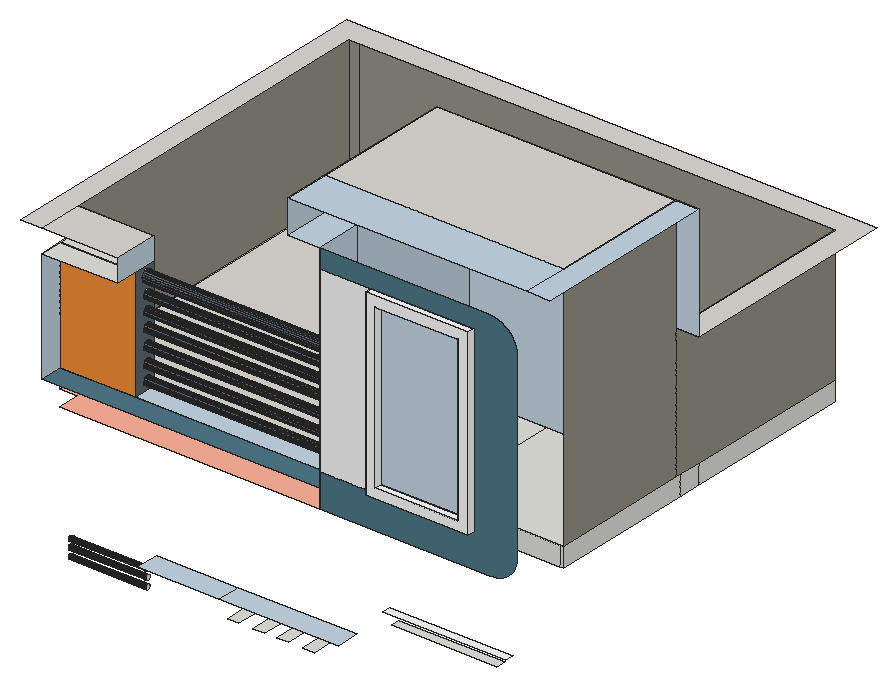
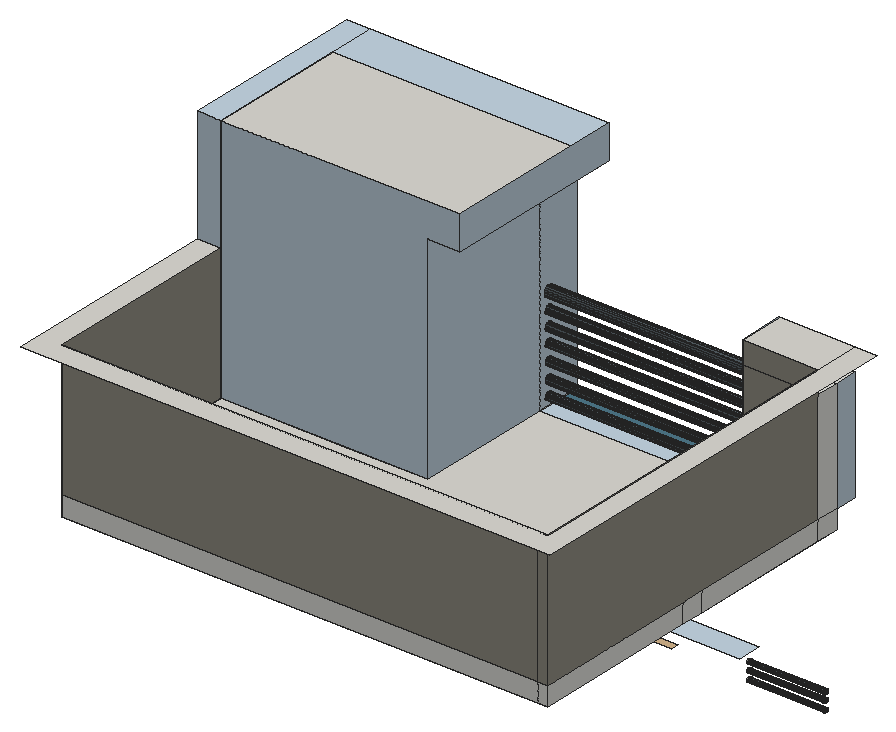
# SketchUp Ruby script. Lengths in inches.
U = 1.inch
M = Sketchup.active_model
def pt(a) = Geom::Point3d.new(a.map { |v| v * U })
def face(e, loops, mat)
  f = e.add_face(loops[0].map { |a| pt(a) })
  loops[1..].each { |l| e.add_face(l.map { |a| pt(a) }).erase! }
  f.material = f.back_material = mat if mat
  f
end
# faces: each face lists its corners as indices into pts; further lists are holes
def faces(e, pts, list, mat = nil) = list.each { |f| face(e, (f[0].is_a?(Array) ? f : [f]).map { |l| l.map { |i| pts[i] } }, mat) }
# xy, xz, yz: faces in a plane at the given z, y or x. An outline is a flat list of corners, or four numbers for a rectangle; further outlines are holes
def ring(l) = l.size == 4 ? [[l[0], l[1]], [l[2], l[1]], [l[2], l[3]], [l[0], l[3]]] : l.each_slice(2).to_a
def flat(e, list, mat, &to3) = list.each { |f| face(e, (f[0].is_a?(Array) ? f : [f]).map { |l| ring(l).map { |u, v| to3.(u, v) } }, mat) }
def xy(e, z, list, mat = nil) = flat(e, list, mat) { |x, y| [x, y, z] }
def xz(e, y, list, mat = nil) = flat(e, list, mat) { |x, z| [x, y, z] }
def yz(e, x, list, mat = nil) = flat(e, list, mat) { |y, z| [x, y, z] }
def lines(e, pts, list) = list.each { |a, b| e.add_line(pt(pts[a]), pt(pts[b])) }
# prism: a flat outline (further loops are holes) pulled along v
def prism(e, loops, v, mat = nil)
  f = face(e, loops, mat); d = Geom::Vector3d.new(v.map { |x| x * U })
  f.pushpull(f.normal.samedirection?(d) ? d.length : -d.length)
end
def box(e, o, s, mat = nil) = prism(e, [[o, [o[0] + s[0], o[1], o[2]], [o[0] + s[0], o[1] + s[1], o[2]], [o[0], o[1] + s[1], o[2]]]], [0, 0, s[2]], mat)
def at(x, y, z, deg = 0) = Geom::Transformation.translation(pt([x, y, z])) * Geom::Transformation.rotation(ORIGIN, Z_AXIS, deg.degrees)
def axes(o, x, y, z) = Geom::Transformation.new([*x, 0, *y, 0, *z, 0, *pt(o).to_a, 1])
def part(name) = M.definitions.add(name)
# library, detail: a bought-in or finely detailed component or shape, given as its bounding box
def library(name, o, s) = part(name).tap { |d| box(d.entities, o, s) }
def detail(e, o, s) = box(e.add_group.entities, o, s)
def put(e, d, t, mat = nil) = e.add_instance(d, t).tap { |i| i.material = mat if mat }
def group(e, t, mat = nil) = e.add_group.tap { |g| g.transformation = t; g.material = mat if mat }.entities
root = M.entities
M.materials.add("[0035_Tan]").color = [210, 180, 140]
M.materials.add("[0096_SkyBlue]").color = [79, 120, 137]
M.materials.add("[Blinds Vertical Pattern]").color = [247, 247, 249]
M.materials.add("[Cladding Siding Tan]").color = [242, 141, 55]
M.materials.add("[Color B02]").color = [255, 178, 153]
M.materials.add("[Formica Graystone]").color = [149, 146, 135]
M.materials.add("[Formica Speckled Grey]").color = [94, 105, 111]
M.materials.add("[Quartz Light Grey]").color = [251, 251, 252]
M.materials.add("[Terrazzo Light Blue]").color = [196, 214, 227]
M.materials.add("[Terrazzo Tile Light]").color = [219, 217, 210]
xy(root,314.29,[[158.09,175.18,164.38,187.5],[171.84,175.18,178.13,187.5],[184.46,175.18,190.75,187.5],[198.34,175.18,204.63,187.5]])
xy(root,322.125,[[110.1875,175.18,153.69,187.5],[153.69,175.18,217.34,187.5]],"[Terrazzo Light Blue]")
xy(root,354.33,[[259.5625,157.81,315.92,162.87]])
xy(root,358.97,[[254.93,157.81,320.55,162.87]],"[Quartz Light Grey]")
xy(root,372.97,[[81.24,265.26,131.93,269.39]],"[0035_Tan]")
xy(root,375.1875,[[158.92,265.26,207.48,270.7]],"[0035_Tan]")
xy(root,392.8125,[[68.53,265.26,328.05,277.89],[68.53,277.89,328.05,368.29]])
xy(root,392.8125,[[78.16,162.87,78.16,175.18,68.53,175.18,68.53,265.26,328.05,265.26,328.05,187.5,217.34,187.5,217.34,162.87]],"[Color B02]")
xy(root,403.0625,[[68.53,175.18,109.08,187.5],[217.34,187.5,259.37,262.25],[259.37,187.5,328.05,262.25]])
xy(root,403.0625,[[68.53,162.87,217.34,175.18]],"[0096_SkyBlue]")
xy(root,403.0625,[[109.08,175.18,217.34,187.5]],"[Terrazzo Light Blue]")
xy(root,403.0625,[[68.53,187.5,217.34,187.5,217.34,262.25,328.05,262.25,328.05,368.29,68.53,368.29]],"[Terrazzo Tile Light]")
xy(root,410.86,[[244.72,159.06,299.47,162.87]],"[Quartz Light Grey]")
xy(root,416.07,[[249.93,159.06,294.25,162.87]],"[Quartz Light Grey]")
xy(root,463,[[68.53,162.87,109.08,175.18],[68.53,175.18,109.08,187.5]])
xy(root,475.0625,[[57.16,162.87,68.53,162.87,68.53,368.29,328.05,368.29,328.05,262.25,340.49,262.25,340.49,380.73,57.16,380.73],[68.53,162.87,109.08,187.5]],"[Terrazzo Tile Light]")
xy(root,502.83,[[249.93,159.06,294.25,162.87]],"[Quartz Light Grey]")
xy(root,508.05,[[244.72,159.06,299.47,162.87]],"[Quartz Light Grey]")
xy(root,518.04,[[200.4,162.87,217.34,262.25]],"[Terrazzo Light Blue]")
xy(root,536.0625,[[200.4,162.87,328.05,187.5],[328.05,162.87,340.49,262.25]],"[Terrazzo Light Blue]")
xy(root,536.0625,[[200.4,187.5,328.05,262.25]],"[Terrazzo Tile Light]")
xz(root,159.06,[[[244.72,410.86,299.47,508.05],[249.93,416.07,294.25,502.83]]],"[Quartz Light Grey]")
xz(root,162.87,[[[244.72,410.86,299.47,508.05],[249.93,416.07,294.25,502.83]]])
xz(root,162.87,[[217.34,392.8125,308.15,392.8125,310.0625,392.92,311.9375,393.25,313.75,393.78,315.47,394.52,317.06,395.44,318.5,396.54,319.76,397.79,320.82,399.17,321.67,400.66,322.28,402.24,322.65,403.87,322.78,405.53,322.78,503.56,322.64,505.45,322.21,507.31,321.51,509.1,320.55,510.8,319.34,512.375,317.9,513.8,316.26,515.05,314.45,516.1,312.5,516.9375,310.4375,517.55,308.3,517.92,306.125,518.04,217.34,518.04,217.34,508.05,299.47,508.05,299.47,410.86,217.34,410.86]],"[0096_SkyBlue]")
xz(root,162.87,[[217.34,410.86,244.72,508.05]],"[Blinds Vertical Pattern]")
xz(root,162.87,[[249.93,416.07,294.25,502.83]],"[Terrazzo Light Blue]")
xz(root,175.18,[[68.53,403.0625,109.08,463]],"[Cladding Siding Tan]")
xz(root,187.5,[[217.34,392.8125,259.37,403.0625],[259.37,392.8125,326.14,403.0625],[326.14,392.8125,328.05,403.0625]])
xz(root,187.5,[[68.53,403.0625,109.08,463],[68.53,463,109.08,475.0625]],"[Formica Graystone]")
xz(root,262.25,[[217.34,403.0625,217.34,518.04,200.4,518.04,200.4,536.0625,328.05,536.0625,328.05,403.0625],[328.05,475.0625,340.49,536.0625]],"[Terrazzo Light Blue]")
xz(root,368.29,[[68.53,392.8125,73.72,403.0625],[73.72,392.8125,328.05,403.0625]])
xz(root,368.29,[[68.53,403.0625,73.72,475.0625],[73.72,403.0625,328.05,475.0625]],"[Formica Graystone]")
yz(root,68.53,[[175.18,392.8125,187.5,403.0625],[187.5,392.8125,265.26,403.0625],[265.26,392.8125,277.89,403.0625],[277.89,392.8125,368.29,403.0625],[175.18,403.0625,187.5,463]])
yz(root,68.53,[[187.5,403.0625,368.29,475.0625]],"[Formica Graystone]")
yz(root,68.53,[[162.87,403.0625,175.18,463]],"[Terrazzo Light Blue]")
yz(root,109.08,[[182.31,406.04,181.76,406.12,181.24,406.33,180.8,406.67,180.47,407.11,180.25,407.62,180.18,408.17,180.25,408.72,180.47,409.23,180.8,409.67,181.24,410.01,181.76,410.22,182.31,410.29,182.86,410.22,183.37,410.01,183.81,409.67,184.15,409.23,184.36,408.72,184.43,408.17,184.36,407.62,184.15,407.11,183.81,406.67,183.37,406.33,182.86,406.12],[182.31,414.11,181.76,414.18,181.24,414.39,180.8,414.73,180.47,415.17,180.25,415.68,180.18,416.23,180.25,416.78,180.47,417.29,180.8,417.73,181.24,418.07,181.76,418.28,182.31,418.36,182.86,418.28,183.37,418.07,183.81,417.73,184.15,417.29,184.36,416.78,184.43,416.23,184.36,415.68,184.15,415.17,183.81,414.73,183.37,414.39,182.86,414.18],[182.31,422.73,181.76,422.8,181.24,423.02,180.8,423.35,180.47,423.79,180.25,424.31,180.18,424.86,180.25,425.41,180.47,425.92,180.8,426.36,181.24,426.7,181.76,426.91,182.31,426.98,182.86,426.91,183.37,426.7,183.81,426.36,184.15,425.92,184.36,425.41,184.43,424.86,184.36,424.31,184.15,423.79,183.81,423.35,183.37,423.02,182.86,422.8],[182.31,431.42,181.76,431.49,181.24,431.7,180.8,432.04,180.47,432.48,180.25,432.99,180.18,433.54,180.25,434.09,180.47,434.61,180.8,435.05,181.24,435.39,181.76,435.6,182.31,435.67,182.86,435.6,183.37,435.39,183.81,435.05,184.15,434.61,184.36,434.09,184.43,433.54,184.36,432.99,184.15,432.48,183.81,432.04,183.37,431.7,182.86,431.49],[182.31,439.29,181.76,439.37,181.24,439.58,180.8,439.92,180.47,440.36,180.25,440.87,180.18,441.42,180.25,441.97,180.47,442.48,180.8,442.92,181.24,443.26,181.76,443.47,182.31,443.54,182.86,443.47,183.37,443.26,183.81,442.92,184.15,442.48,184.36,441.97,184.43,441.42,184.36,440.87,184.15,440.36,183.81,439.92,183.37,439.58,182.86,439.37],
  [182.31,447.36,181.76,447.43,181.24,447.64,180.8,447.98,180.47,448.42,180.25,448.93,180.18,449.48,180.25,450.03,180.47,450.54,180.8,450.98,181.24,451.32,181.76,451.53,182.31,451.61,182.86,451.53,183.37,451.32,183.81,450.98,184.15,450.54,184.36,450.03,184.43,449.48,184.36,448.93,184.15,448.42,183.81,447.98,183.37,447.64,182.86,447.43],[181.99,455.25,181.19,455.36,180.45,455.66,179.82,456.15,179.33,456.78,179.03,457.52,178.92,458.3125,179.03,459.11,179.33,459.85,179.82,460.48,180.45,460.97,181.19,461.27,181.99,461.375,182.78,461.27,183.52,460.97,184.15,460.48,184.64,459.85,184.94,459.11,185.05,458.3125,184.94,457.52,184.64,456.78,184.15,456.15,183.52,455.66,182.78,455.36]])
yz(root,109.08,[[[175.18,403.0625,187.5,463],[181.99,455.25,181.19,455.36,180.45,455.66,179.82,456.15,179.33,456.78,179.03,457.52,178.92,458.3125,179.03,459.11,179.33,459.85,179.82,460.48,180.45,460.97,181.19,461.27,181.99,461.375,182.78,461.27,183.52,460.97,184.15,460.48,184.64,459.85,184.94,459.11,185.05,458.3125,184.94,457.52,184.64,456.78,184.15,456.15,183.52,455.66,182.78,455.36],[182.31,447.36,181.76,447.43,181.24,447.64,180.8,447.98,180.47,448.42,180.25,448.93,180.18,449.48,180.25,450.03,180.47,450.54,180.8,450.98,181.24,451.32,181.76,451.53,182.31,451.61,182.86,451.53,183.37,451.32,183.81,450.98,184.15,450.54,184.36,450.03,184.43,449.48,184.36,448.93,184.15,448.42,183.81,447.98,183.37,447.64,182.86,447.43],[182.31,406.04,181.76,406.12,181.24,406.33,180.8,406.67,180.47,407.11,180.25,407.62,180.18,408.17,180.25,408.72,180.47,409.23,180.8,409.67,181.24,410.01,181.76,410.22,182.31,410.29,182.86,410.22,183.37,410.01,183.81,409.67,184.15,409.23,184.36,408.72,184.43,408.17,184.36,407.62,184.15,407.11,183.81,406.67,183.37,406.33,182.86,406.12],[182.31,439.29,181.76,439.37,181.24,439.58,180.8,439.92,180.47,440.36,180.25,440.87,180.18,441.42,180.25,441.97,180.47,442.48,180.8,442.92,181.24,443.26,181.76,443.47,182.31,443.54,182.86,443.47,183.37,443.26,183.81,442.92,184.15,442.48,184.36,441.97,184.43,441.42,184.36,440.87,184.15,440.36,183.81,439.92,183.37,439.58,182.86,439.37],[182.31,414.11,181.76,414.18,181.24,414.39,180.8,414.73,180.47,415.17,180.25,415.68,180.18,416.23,180.25,416.78,180.47,417.29,180.8,417.73,181.24,418.07,181.76,418.28,182.31,418.36,182.86,418.28,183.37,418.07,183.81,417.73,184.15,417.29,184.36,416.78,184.43,416.23,184.36,415.68,184.15,415.17,183.81,414.73,183.37,414.39,182.86,414.18],[182.31,431.42,181.76,431.49,181.24,431.7,180.8,432.04,180.47,432.48,180.25,432.99,180.18,433.54,180.25,434.09,180.47,434.61,180.8,435.05,181.24,435.39,181.76,435.6,182.31,435.67,182.86,435.6,183.37,435.39,183.81,435.05,184.15,434.61,184.36,434.09,184.43,433.54,184.36,432.99,184.15,432.48,183.81,432.04,183.37,431.7,182.86,431.49],[182.31,422.73,181.76,422.8,181.24,423.02,180.8,423.35,180.47,423.79,180.25,424.31,180.18,424.86,180.25,425.41,180.47,425.92,180.8,426.36,181.24,426.7,181.76,426.91,182.31,426.98,182.86,426.91,183.37,426.7,183.81,426.36,184.15,425.92,184.36,425.41,184.43,424.86,184.36,424.31,184.15,423.79,183.81,423.35,183.37,423.02,182.86,422.8]]],"[Formica Speckled Grey]")
yz(root,109.08,[[162.87,463,187.5,475.0625]],"[Terrazzo Light Blue]")
yz(root,110.1875,[[181.95,308.5,182.24,308.53,182.51,308.65,182.75,308.83,182.93,309.06,183.04,309.33,183.08,309.62,183.04,309.91,182.93,310.18,182.75,310.42,182.51,310.6,182.24,310.71,181.95,310.75,181.66,310.71,181.39,310.6,181.16,310.42,180.98,310.18,180.86,309.91,180.83,309.62,180.86,309.33,180.98,309.06,181.16,308.83,181.39,308.65,181.66,308.53],[181.95,313,182.24,313.03,182.51,313.15,182.75,313.33,182.93,313.56,183.04,313.83,183.08,314.12,183.04,314.41,182.93,314.68,182.75,314.92,182.51,315.1,182.24,315.21,181.95,315.25,181.66,315.21,181.39,315.1,181.16,314.92,180.98,314.68,180.86,314.41,180.83,314.12,180.86,313.83,180.98,313.56,181.16,313.33,181.39,313.15,181.66,313.03],[181.95,317.18,182.24,317.22,182.51,317.33,182.75,317.51,182.93,317.75,183.04,318.02,183.08,318.31,183.04,318.6,182.93,318.87,182.75,319.1,182.51,319.28,182.24,319.4,181.95,319.43,181.66,319.4,181.39,319.28,181.16,319.1,180.98,318.87,180.86,318.6,180.83,318.31,180.86,318.02,180.98,317.75,181.16,317.51,181.39,317.33,181.66,317.22]])
yz(root,200.4,[[162.87,518.04,262.25,536.0625]],"[Terrazzo Light Blue]")
yz(root,217.34,[[162.87,392.8125,187.5,403.0625]])
yz(root,217.34,[[[162.87,403.0625,187.5,518.04],[181.99,455.25,182.78,455.36,183.52,455.66,184.15,456.15,184.64,456.78,184.94,457.52,185.05,458.3125,184.94,459.11,184.64,459.85,184.15,460.48,183.52,460.97,182.78,461.27,181.99,461.375,181.19,461.27,180.45,460.97,179.82,460.48,179.33,459.85,179.03,459.11,178.92,458.3125,179.03,457.52,179.33,456.78,179.82,456.15,180.45,455.66,181.19,455.36],[182.31,406.04,182.86,406.12,183.37,406.33,183.81,406.67,184.15,407.11,184.36,407.62,184.43,408.17,184.36,408.72,184.15,409.23,183.81,409.67,183.37,410.01,182.86,410.22,182.31,410.29,181.76,410.22,181.24,410.01,180.8,409.67,180.47,409.23,180.25,408.72,180.18,408.17,180.25,407.62,180.47,407.11,180.8,406.67,181.24,406.33,181.76,406.12],[182.31,414.11,182.86,414.18,183.37,414.39,183.81,414.73,184.15,415.17,184.36,415.68,184.43,416.23,184.36,416.78,184.15,417.29,183.81,417.73,183.37,418.07,182.86,418.28,182.31,418.36,181.76,418.28,181.24,418.07,180.8,417.73,180.47,417.29,180.25,416.78,180.18,416.23,180.25,415.68,180.47,415.17,180.8,414.73,181.24,414.39,181.76,414.18],[182.31,422.73,182.86,422.8,183.37,423.02,183.81,423.35,184.15,423.79,184.36,424.31,184.43,424.86,184.36,425.41,184.15,425.92,183.81,426.36,183.37,426.7,182.86,426.91,182.31,426.98,181.76,426.91,181.24,426.7,180.8,426.36,180.47,425.92,180.25,425.41,180.18,424.86,180.25,424.31,180.47,423.79,180.8,423.35,181.24,423.02,181.76,422.8],[182.31,431.42,182.86,431.49,183.37,431.7,183.81,432.04,184.15,432.48,184.36,432.99,184.43,433.54,184.36,434.09,184.15,434.61,183.81,435.05,183.37,435.39,182.86,435.6,182.31,435.67,181.76,435.6,181.24,435.39,180.8,435.05,180.47,434.61,180.25,434.09,180.18,433.54,180.25,432.99,180.47,432.48,180.8,432.04,181.24,431.7,181.76,431.49],[182.31,439.29,182.86,439.37,183.37,439.58,183.81,439.92,184.15,440.36,184.36,440.87,184.43,441.42,184.36,441.97,184.15,442.48,183.81,442.92,183.37,443.26,182.86,443.47,182.31,443.54,181.76,443.47,181.24,443.26,180.8,442.92,180.47,442.48,180.25,441.97,180.18,441.42,180.25,440.87,180.47,440.36,180.8,439.92,181.24,439.58,181.76,439.37],[182.31,447.36,182.86,447.43,183.37,447.64,183.81,447.98,184.15,448.42,184.36,448.93,184.43,449.48,184.36,450.03,184.15,450.54,183.81,450.98,183.37,451.32,182.86,451.53,182.31,451.61,181.76,451.53,181.24,451.32,180.8,450.98,180.47,450.54,180.25,450.03,180.18,449.48,180.25,448.93,180.47,448.42,180.8,447.98,181.24,447.64,181.76,447.43]],[187.5,403.0625,262.25,518.04]],"[Terrazzo Light Blue]")
yz(root,244.72,[[159.06,410.86,162.87,508.05]],"[Quartz Light Grey]")
yz(root,249.93,[[159.06,416.07,162.87,502.83]],"[Quartz Light Grey]")
yz(root,294.25,[[159.06,416.07,162.87,502.83]],"[Quartz Light Grey]")
yz(root,299.47,[[159.06,410.86,162.87,508.05]],"[Quartz Light Grey]")
yz(root,328.05,[[187.5,392.8125,265.26,403.0625],[265.26,392.8125,277.89,403.0625],[277.89,392.8125,368.29,403.0625]])
yz(root,328.05,[[187.5,403.0625,262.25,536.0625],[262.25,403.0625,368.29,475.0625]],"[Formica Graystone]")
p = [[110.1875,181.66,308.53],[110.1875,181.39,308.65],[68.53,181.39,308.65],[68.53,181.66,308.53],[110.1875,181.95,308.5],[68.53,181.95,308.5],
  [110.1875,182.24,308.53],[68.53,182.24,308.53],[110.1875,182.51,308.65],[68.53,182.51,308.65],[110.1875,181.16,308.83],[68.53,181.16,308.83],
  [110.1875,182.75,308.83],[68.53,182.75,308.83],[110.1875,180.98,309.06],[68.53,180.98,309.06],[110.1875,182.93,309.06],[68.53,182.93,309.06],
  [110.1875,180.86,309.33],[68.53,180.86,309.33],[110.1875,183.04,309.33],[68.53,183.04,309.33],[110.1875,180.83,309.62],[68.53,180.83,309.62],
  [110.1875,183.08,309.62],[68.53,183.08,309.62],[110.1875,180.86,309.91],[68.53,180.86,309.91],[110.1875,183.04,309.91],[68.53,183.04,309.91],
  [110.1875,180.98,310.18],[68.53,180.98,310.18],[110.1875,182.93,310.18],[68.53,182.93,310.18],[110.1875,181.16,310.42],[68.53,181.16,310.42],
  [110.1875,182.75,310.42],[68.53,182.75,310.42],[110.1875,181.39,310.6],[68.53,181.39,310.6],[110.1875,182.51,310.6],[68.53,182.51,310.6],
  [110.1875,181.66,310.71],[68.53,181.66,310.71],[110.1875,182.24,310.71],[68.53,182.24,310.71],[110.1875,181.95,310.75],[68.53,181.95,310.75],
  [110.1875,181.66,313.03],[110.1875,181.39,313.15],[68.53,181.39,313.15],[68.53,181.66,313.03],[110.1875,181.95,313],[68.53,181.95,313],
  [110.1875,182.24,313.03],[68.53,182.24,313.03],[110.1875,182.51,313.15],[68.53,182.51,313.15],[110.1875,181.16,313.33],[68.53,181.16,313.33],
  [110.1875,182.75,313.33],[68.53,182.75,313.33],[110.1875,180.98,313.56],[68.53,180.98,313.56],[110.1875,182.93,313.56],[68.53,182.93,313.56],
  [110.1875,180.86,313.83],[68.53,180.86,313.83],[110.1875,183.04,313.83],[68.53,183.04,313.83],[110.1875,180.83,314.12],[68.53,180.83,314.12],
  [110.1875,183.08,314.12],[68.53,183.08,314.12],[110.1875,180.86,314.41],[68.53,180.86,314.41],[110.1875,183.04,314.41],[68.53,183.04,314.41],
  [110.1875,180.98,314.68],[68.53,180.98,314.68],[110.1875,182.93,314.68],[68.53,182.93,314.68],[110.1875,181.16,314.92],[68.53,181.16,314.92],
  [110.1875,182.75,314.92],[68.53,182.75,314.92],[110.1875,181.39,315.1],[68.53,181.39,315.1],[110.1875,182.51,315.1],[68.53,182.51,315.1],
  [110.1875,181.66,315.21],[68.53,181.66,315.21],[110.1875,182.24,315.21],[68.53,182.24,315.21],[110.1875,181.95,315.25],[68.53,181.95,315.25],
  [110.1875,181.66,317.22],[110.1875,181.39,317.33],[68.53,181.39,317.33],[68.53,181.66,317.22],[110.1875,181.95,317.18],[68.53,181.95,317.18],
  [110.1875,182.24,317.22],[68.53,182.24,317.22],[110.1875,182.51,317.33],[68.53,182.51,317.33],[110.1875,181.16,317.51],[68.53,181.16,317.51],
  [110.1875,182.75,317.51],[68.53,182.75,317.51],[110.1875,180.98,317.75],[68.53,180.98,317.75],[110.1875,182.93,317.75],[68.53,182.93,317.75],
  [110.1875,180.86,318.02],[68.53,180.86,318.02],[110.1875,183.04,318.02],[68.53,183.04,318.02],[110.1875,180.83,318.31],[68.53,180.83,318.31],
  [110.1875,183.08,318.31],[68.53,183.08,318.31],[110.1875,180.86,318.6],[68.53,180.86,318.6],[110.1875,183.04,318.6],[68.53,183.04,318.6],
  [110.1875,180.98,318.87],[68.53,180.98,318.87],[110.1875,182.93,318.87],[68.53,182.93,318.87],[110.1875,181.16,319.1],[68.53,181.16,319.1],
  [110.1875,182.75,319.1],[68.53,182.75,319.1],[110.1875,181.39,319.28],[68.53,181.39,319.28],[110.1875,182.51,319.28],[68.53,182.51,319.28],
  [110.1875,181.66,319.4],[68.53,181.66,319.4],[110.1875,182.24,319.4],[68.53,182.24,319.4],[110.1875,181.95,319.43],[68.53,181.95,319.43],
  [109.08,181.76,406.12],[109.08,182.31,406.04],[217.34,182.31,406.04],[217.34,181.76,406.12],[109.08,182.86,406.12],[217.34,182.86,406.12],
  [109.08,181.24,406.33],[217.34,181.24,406.33],[109.08,183.37,406.33],[217.34,183.37,406.33],[109.08,180.8,406.67],[217.34,180.8,406.67],
  [109.08,183.81,406.67],[217.34,183.81,406.67],[109.08,180.47,407.11],[217.34,180.47,407.11],[109.08,184.15,407.11],[217.34,184.15,407.11],
  [109.08,180.25,407.62],[217.34,180.25,407.62],[109.08,184.36,407.62],[217.34,184.36,407.62],[109.08,180.18,408.17],[217.34,180.18,408.17],
  [109.08,184.43,408.17],[217.34,184.43,408.17],[109.08,180.25,408.72],[217.34,180.25,408.72],[109.08,184.36,408.72],[217.34,184.36,408.72],
  [109.08,180.47,409.23],[217.34,180.47,409.23],[109.08,184.15,409.23],[217.34,184.15,409.23],[109.08,180.8,409.67],[217.34,180.8,409.67],
  [109.08,183.81,409.67],[217.34,183.81,409.67],[109.08,181.24,410.01],[217.34,181.24,410.01],[109.08,183.37,410.01],[217.34,183.37,410.01],
  [109.08,181.76,410.22],[217.34,181.76,410.22],[109.08,182.86,410.22],[217.34,182.86,410.22],[109.08,182.31,410.29],[217.34,182.31,410.29],
  [109.08,181.76,414.18],[109.08,182.31,414.11],[217.34,182.31,414.11],[217.34,181.76,414.18],[109.08,182.86,414.18],[217.34,182.86,414.18],
  [109.08,181.24,414.39],[217.34,181.24,414.39],[109.08,183.37,414.39],[217.34,183.37,414.39],[109.08,180.8,414.73],[217.34,180.8,414.73],
  [109.08,183.81,414.73],[217.34,183.81,414.73],[109.08,180.47,415.17],[217.34,180.47,415.17],[109.08,184.15,415.17],[217.34,184.15,415.17],
  [109.08,180.25,415.68],[217.34,180.25,415.68],[109.08,184.36,415.68],[217.34,184.36,415.68],[109.08,180.18,416.23],[217.34,180.18,416.23],
  [109.08,184.43,416.23],[217.34,184.43,416.23],[109.08,180.25,416.78],[217.34,180.25,416.78],[109.08,184.36,416.78],[217.34,184.36,416.78],
  [109.08,180.47,417.29],[217.34,180.47,417.29],[109.08,184.15,417.29],[217.34,184.15,417.29],[109.08,180.8,417.73],[217.34,180.8,417.73],
  [109.08,183.81,417.73],[217.34,183.81,417.73],[109.08,181.24,418.07],[217.34,181.24,418.07],[109.08,183.37,418.07],[217.34,183.37,418.07],
  [109.08,181.76,418.28],[217.34,181.76,418.28],[109.08,182.86,418.28],[217.34,182.86,418.28],[109.08,182.31,418.36],[217.34,182.31,418.36],
  [109.08,181.76,422.8],[109.08,182.31,422.73],[217.34,182.31,422.73],[217.34,181.76,422.8],[109.08,182.86,422.8],[217.34,182.86,422.8],
  [109.08,181.24,423.02],[217.34,181.24,423.02],[109.08,183.37,423.02],[217.34,183.37,423.02],[109.08,180.8,423.35],[217.34,180.8,423.35],
  [109.08,183.81,423.35],[217.34,183.81,423.35],[109.08,180.47,423.79],[217.34,180.47,423.79],[109.08,184.15,423.79],[217.34,184.15,423.79],
  [109.08,180.25,424.31],[217.34,180.25,424.31],[109.08,184.36,424.31],[217.34,184.36,424.31],[109.08,180.18,424.86],[217.34,180.18,424.86],
  [109.08,184.43,424.86],[217.34,184.43,424.86],[109.08,180.25,425.41],[217.34,180.25,425.41],[109.08,184.36,425.41],[217.34,184.36,425.41],
  [109.08,180.47,425.92],[217.34,180.47,425.92],[109.08,184.15,425.92],[217.34,184.15,425.92],[109.08,180.8,426.36],[217.34,180.8,426.36],
  [109.08,183.81,426.36],[217.34,183.81,426.36],[109.08,181.24,426.7],[217.34,181.24,426.7],[109.08,183.37,426.7],[217.34,183.37,426.7],
  [109.08,181.76,426.91],[217.34,181.76,426.91],[109.08,182.86,426.91],[217.34,182.86,426.91],[109.08,182.31,426.98],[217.34,182.31,426.98],
  [109.08,181.76,431.49],[109.08,182.31,431.42],[217.34,182.31,431.42],[217.34,181.76,431.49],[109.08,182.86,431.49],[217.34,182.86,431.49],
  [109.08,181.24,431.7],[217.34,181.24,431.7],[109.08,183.37,431.7],[217.34,183.37,431.7],[109.08,180.8,432.04],[217.34,180.8,432.04],
  [109.08,183.81,432.04],[217.34,183.81,432.04],[109.08,180.47,432.48],[217.34,180.47,432.48],[109.08,184.15,432.48],[217.34,184.15,432.48],
  [109.08,180.25,432.99],[217.34,180.25,432.99],[109.08,184.36,432.99],[217.34,184.36,432.99],[109.08,180.18,433.54],[217.34,180.18,433.54],
  [109.08,184.43,433.54],[217.34,184.43,433.54],[109.08,180.25,434.09],[217.34,180.25,434.09],[109.08,184.36,434.09],[217.34,184.36,434.09],
  [109.08,180.47,434.61],[217.34,180.47,434.61],[109.08,184.15,434.61],[217.34,184.15,434.61],[109.08,180.8,435.05],[217.34,180.8,435.05],
  [109.08,183.81,435.05],[217.34,183.81,435.05],[109.08,181.24,435.39],[217.34,181.24,435.39],[109.08,183.37,435.39],[217.34,183.37,435.39],
  [109.08,181.76,435.6],[217.34,181.76,435.6],[109.08,182.86,435.6],[217.34,182.86,435.6],[109.08,182.31,435.67],[217.34,182.31,435.67],
  [109.08,181.76,439.37],[109.08,182.31,439.29],[217.34,182.31,439.29],[217.34,181.76,439.37],[109.08,182.86,439.37],[217.34,182.86,439.37],
  [109.08,181.24,439.58],[217.34,181.24,439.58],[109.08,183.37,439.58],[217.34,183.37,439.58],[109.08,180.8,439.92],[217.34,180.8,439.92],
  [109.08,183.81,439.92],[217.34,183.81,439.92],[109.08,180.47,440.36],[217.34,180.47,440.36],[109.08,184.15,440.36],[217.34,184.15,440.36],
  [109.08,180.25,440.87],[217.34,180.25,440.87],[109.08,184.36,440.87],[217.34,184.36,440.87],[109.08,180.18,441.42],[217.34,180.18,441.42],
  [109.08,184.43,441.42],[217.34,184.43,441.42],[109.08,180.25,441.97],[217.34,180.25,441.97],[109.08,184.36,441.97],[217.34,184.36,441.97],
  [109.08,180.47,442.48],[217.34,180.47,442.48],[109.08,184.15,442.48],[217.34,184.15,442.48],[109.08,180.8,442.92],[217.34,180.8,442.92],
  [109.08,183.81,442.92],[217.34,183.81,442.92],[109.08,181.24,443.26],[217.34,181.24,443.26],[109.08,183.37,443.26],[217.34,183.37,443.26],
  [109.08,181.76,443.47],[217.34,181.76,443.47],[109.08,182.86,443.47],[217.34,182.86,443.47],[109.08,182.31,443.54],[217.34,182.31,443.54],
  [109.08,181.24,447.64],[109.08,181.76,447.43],[217.34,181.76,447.43],[217.34,181.24,447.64],[109.08,182.31,447.36],[217.34,182.31,447.36],
  [109.08,182.86,447.43],[217.34,182.86,447.43],[109.08,183.37,447.64],[217.34,183.37,447.64],[109.08,180.8,447.98],[217.34,180.8,447.98],
  [109.08,183.81,447.98],[217.34,183.81,447.98],[109.08,180.47,448.42],[217.34,180.47,448.42],[109.08,184.15,448.42],[217.34,184.15,448.42],
  [109.08,180.25,448.93],[217.34,180.25,448.93],[109.08,184.36,448.93],[217.34,184.36,448.93],[109.08,180.18,449.48],[217.34,180.18,449.48],
  [109.08,184.43,449.48],[217.34,184.43,449.48],[109.08,180.25,450.03],[217.34,180.25,450.03],[109.08,184.36,450.03],[217.34,184.36,450.03],
  [109.08,180.47,450.54],[217.34,180.47,450.54],[109.08,184.15,450.54],[217.34,184.15,450.54],[109.08,180.8,450.98],[217.34,180.8,450.98],
  [109.08,183.81,450.98],[217.34,183.81,450.98],[109.08,181.24,451.32],[217.34,181.24,451.32],[109.08,183.37,451.32],[217.34,183.37,451.32],
  [109.08,181.76,451.53],[217.34,181.76,451.53],[109.08,182.86,451.53],[217.34,182.86,451.53],[109.08,182.31,451.61],[217.34,182.31,451.61],
  [109.08,181.19,455.36],[109.08,181.99,455.25],[217.34,181.99,455.25],[217.34,181.19,455.36],[109.08,182.78,455.36],[217.34,182.78,455.36],
  [109.08,180.45,455.66],[217.34,180.45,455.66],[109.08,183.52,455.66],[217.34,183.52,455.66],[109.08,179.82,456.15],[217.34,179.82,456.15],
  [109.08,184.15,456.15],[217.34,184.15,456.15],[109.08,179.33,456.78],[217.34,179.33,456.78],[109.08,184.64,456.78],[217.34,184.64,456.78],
  [109.08,179.03,457.52],[217.34,179.03,457.52],[109.08,184.94,457.52],[217.34,184.94,457.52],[109.08,178.92,458.3125],[217.34,178.92,458.3125],
  [109.08,185.05,458.3125],[217.34,185.05,458.3125],[109.08,179.03,459.11],[217.34,179.03,459.11],[109.08,184.94,459.11],[217.34,184.94,459.11],
  [109.08,179.33,459.85],[217.34,179.33,459.85],[109.08,184.64,459.85],[217.34,184.64,459.85],[109.08,179.82,460.48],[217.34,179.82,460.48],
  [109.08,184.15,460.48],[217.34,184.15,460.48],[109.08,180.45,460.97],[217.34,180.45,460.97],[109.08,183.52,460.97],[217.34,183.52,460.97],
  [109.08,181.19,461.27],[217.34,181.19,461.27],[109.08,182.78,461.27],[217.34,182.78,461.27],[109.08,181.99,461.375],[217.34,181.99,461.375]]
faces(root,p,[[0,1,2,3],[4,0,3,5],[6,4,5,7],[8,6,7,9],[1,10,11,2],[12,8,9,13],[10,14,15,11],[16,12,13,17],
  [14,18,19,15],[20,16,17,21],[18,22,23,19],[24,20,21,25],[22,26,27,23],[28,24,25,29],[26,30,31,27],[32,28,29,33],
  [30,34,35,31],[36,32,33,37],[34,38,39,35],[40,36,37,41],[38,42,43,39],[44,40,41,45],[42,46,47,43],[46,44,45,47],
  [48,49,50,51],[52,48,51,53],[54,52,53,55],[56,54,55,57],[49,58,59,50],[60,56,57,61],[58,62,63,59],[64,60,61,65],
  [62,66,67,63],[68,64,65,69],[66,70,71,67],[72,68,69,73],[70,74,75,71],[76,72,73,77],[74,78,79,75],[80,76,77,81],
  [78,82,83,79],[84,80,81,85],[82,86,87,83],[88,84,85,89],[86,90,91,87],[92,88,89,93],[90,94,95,91],[94,92,93,95],
  [96,97,98,99],[100,96,99,101],[102,100,101,103],[104,102,103,105],[97,106,107,98],[108,104,105,109],[106,110,111,107],[112,108,109,113],
  [110,114,115,111],[116,112,113,117],[114,118,119,115],[120,116,117,121],[118,122,123,119],[124,120,121,125],[122,126,127,123],[128,124,125,129],
  [126,130,131,127],[132,128,129,133],[130,134,135,131],[136,132,133,137],[134,138,139,135],[140,136,137,141],[138,142,143,139],[142,140,141,143],
  [144,145,146,147],[145,148,149,146],[150,144,147,151],[148,152,153,149],[154,150,151,155],[152,156,157,153],[158,154,155,159],[156,160,161,157],
  [162,158,159,163],[160,164,165,161],[166,162,163,167],[164,168,169,165],[170,166,167,171],[168,172,173,169],[174,170,171,175],[172,176,177,173],
  [178,174,175,179],[176,180,181,177],[182,178,179,183],[180,184,185,181],[186,182,183,187],[184,188,189,185],[190,186,187,191],[188,190,191,189],
  [192,193,194,195],[193,196,197,194],[198,192,195,199],[196,200,201,197],[202,198,199,203],[200,204,205,201],[206,202,203,207],[204,208,209,205],
  [210,206,207,211],[208,212,213,209],[214,210,211,215],[212,216,217,213],[218,214,215,219],[216,220,221,217],[222,218,219,223],[220,224,225,221],
  [226,222,223,227],[224,228,229,225],[230,226,227,231],[228,232,233,229],[234,230,231,235],[232,236,237,233],[238,234,235,239],[236,238,239,237],
  [240,241,242,243],[241,244,245,242],[246,240,243,247],[244,248,249,245],[250,246,247,251],[248,252,253,249],[254,250,251,255],[252,256,257,253],
  [258,254,255,259],[256,260,261,257],[262,258,259,263],[260,264,265,261],[266,262,263,267],[264,268,269,265],[270,266,267,271],[268,272,273,269],
  [274,270,271,275],[272,276,277,273],[278,274,275,279],[276,280,281,277],[282,278,279,283],[280,284,285,281],[286,282,283,287],[284,286,287,285],
  [288,289,290,291],[289,292,293,290],[294,288,291,295],[292,296,297,293],[298,294,295,299],[296,300,301,297],[302,298,299,303],[300,304,305,301],
  [306,302,303,307],[304,308,309,305],[310,306,307,311],[308,312,313,309],[314,310,311,315],[312,316,317,313],[318,314,315,319],[316,320,321,317],
  [322,318,319,323],[320,324,325,321],[326,322,323,327],[324,328,329,325],[330,326,327,331],[328,332,333,329],[334,330,331,335],[332,334,335,333],
  [336,337,338,339],[337,340,341,338],[342,336,339,343],[340,344,345,341],[346,342,343,347],[344,348,349,345],[350,346,347,351],[348,352,353,349],
  [354,350,351,355],[352,356,357,353],[358,354,355,359],[356,360,361,357],[362,358,359,363],[360,364,365,361],[366,362,363,367],[364,368,369,365],
  [370,366,367,371],[368,372,373,369],[374,370,371,375],[372,376,377,373],[378,374,375,379],[376,380,381,377],[382,378,379,383],[380,382,383,381],
  [384,385,386,387],[385,388,389,386],[388,390,391,389],[390,392,393,391],[394,384,387,395],[392,396,397,393],[398,394,395,399],[396,400,401,397],
  [402,398,399,403],[400,404,405,401],[406,402,403,407],[404,408,409,405],[410,406,407,411],[408,412,413,409],[414,410,411,415],[412,416,417,413],
  [418,414,415,419],[416,420,421,417],[422,418,419,423],[420,424,425,421],[426,422,423,427],[424,428,429,425],[430,426,427,431],[428,430,431,429],
  [432,433,434,435],[433,436,437,434],[438,432,435,439],[436,440,441,437],[442,438,439,443],[440,444,445,441],[446,442,443,447],[444,448,449,445],
  [450,446,447,451],[448,452,453,449],[454,450,451,455],[452,456,457,453],[458,454,455,459],[456,460,461,457],[462,458,459,463],[460,464,465,461],
  [466,462,463,467],[464,468,469,465],[470,466,467,471],[468,472,473,469],[474,470,471,475],[472,476,477,473],[478,474,475,479],[476,478,479,477]],"[Formica Speckled Grey]")
